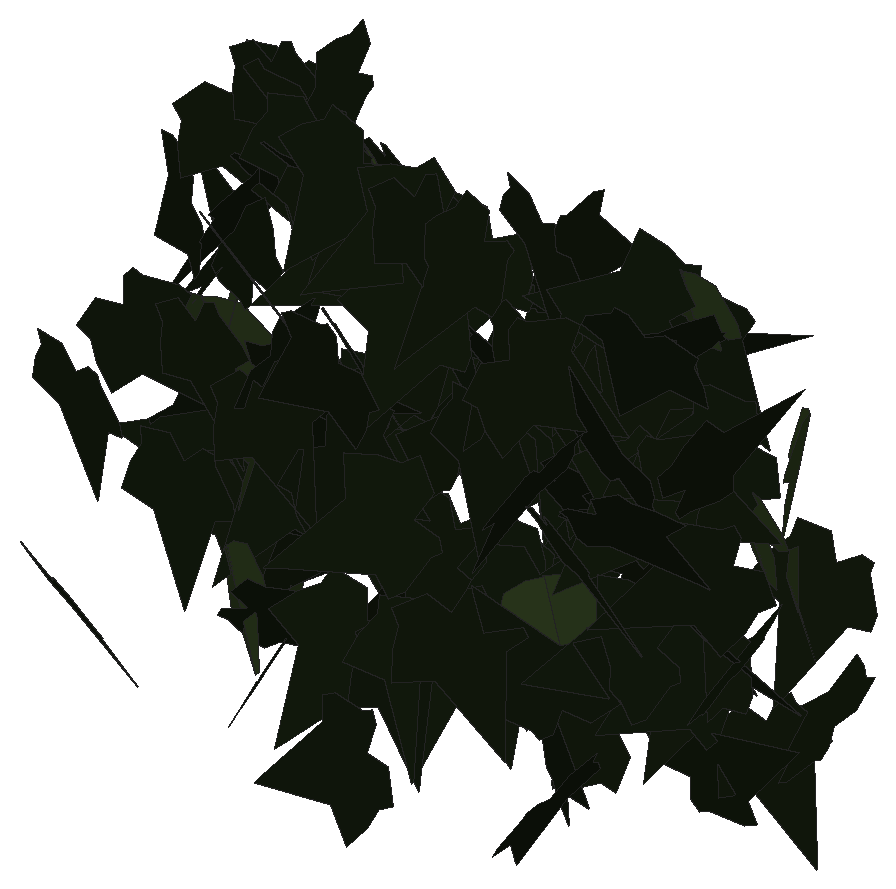
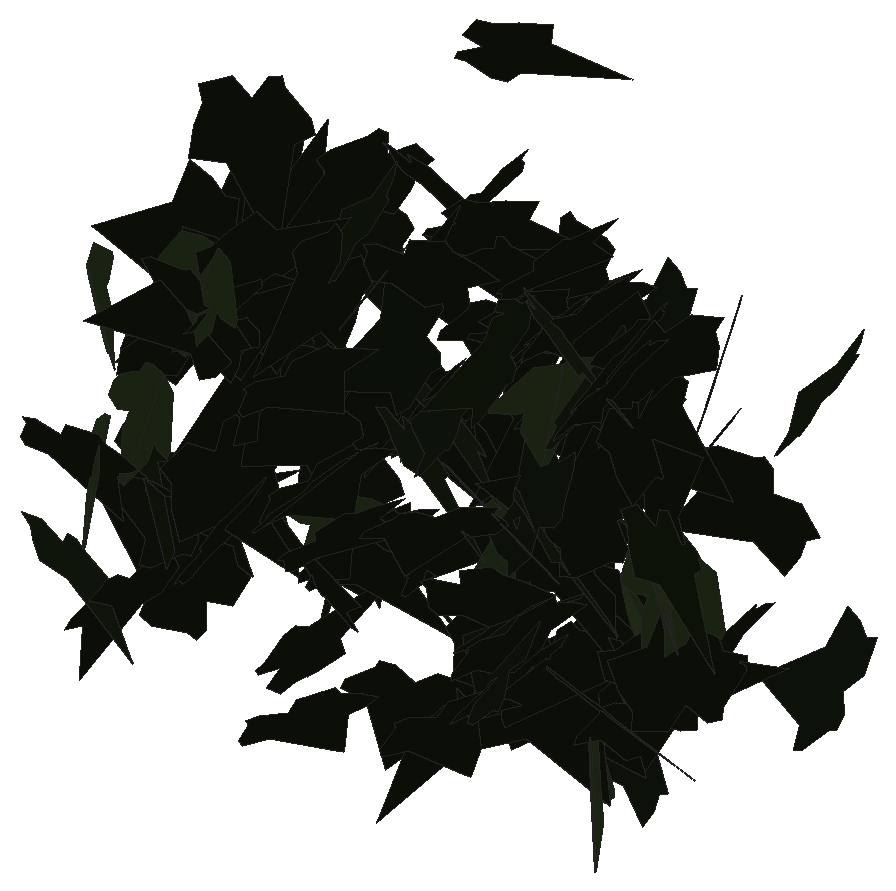
# SketchUp Ruby script. Lengths in inches.
U = 1.inch
M = Sketchup.active_model
def pt(a) = Geom::Point3d.new(a.map { |v| v * U })
def face(e, loops, mat)
  f = e.add_face(loops[0].map { |a| pt(a) })
  loops[1..].each { |l| e.add_face(l.map { |a| pt(a) }).erase! }
  f.material = f.back_material = mat if mat
  f
end
# faces: each face lists its corners as indices into pts; further lists are holes
def faces(e, pts, list, mat = nil) = list.each { |f| face(e, (f[0].is_a?(Array) ? f : [f]).map { |l| l.map { |i| pts[i] } }, mat) }
# xy, xz, yz: faces in a plane at the given z, y or x. An outline is a flat list of corners, or four numbers for a rectangle; further outlines are holes
def ring(l) = l.size == 4 ? [[l[0], l[1]], [l[2], l[1]], [l[2], l[3]], [l[0], l[3]]] : l.each_slice(2).to_a
def flat(e, list, mat, &to3) = list.each { |f| face(e, (f[0].is_a?(Array) ? f : [f]).map { |l| ring(l).map { |u, v| to3.(u, v) } }, mat) }
def xy(e, z, list, mat = nil) = flat(e, list, mat) { |x, y| [x, y, z] }
def xz(e, y, list, mat = nil) = flat(e, list, mat) { |x, z| [x, y, z] }
def yz(e, x, list, mat = nil) = flat(e, list, mat) { |y, z| [x, y, z] }
def lines(e, pts, list) = list.each { |a, b| e.add_line(pt(pts[a]), pt(pts[b])) }
# prism: a flat outline (further loops are holes) pulled along v
def prism(e, loops, v, mat = nil)
  f = face(e, loops, mat); d = Geom::Vector3d.new(v.map { |x| x * U })
  f.pushpull(f.normal.samedirection?(d) ? d.length : -d.length)
end
def box(e, o, s, mat = nil) = prism(e, [[o, [o[0] + s[0], o[1], o[2]], [o[0] + s[0], o[1] + s[1], o[2]], [o[0], o[1] + s[1], o[2]]]], [0, 0, s[2]], mat)
def at(x, y, z, deg = 0) = Geom::Transformation.translation(pt([x, y, z])) * Geom::Transformation.rotation(ORIGIN, Z_AXIS, deg.degrees)
def axes(o, x, y, z) = Geom::Transformation.new([*x, 0, *y, 0, *z, 0, *pt(o).to_a, 1])
def part(name) = M.definitions.add(name)
# library, detail: a bought-in or finely detailed component or shape, given as its bounding box
def library(name, o, s) = part(name).tap { |d| box(d.entities, o, s) }
def detail(e, o, s) = box(e.add_group.entities, o, s)
def put(e, d, t, mat = nil) = e.add_instance(d, t).tap { |i| i.material = mat if mat }
def group(e, t, mat = nil) = e.add_group.tap { |g| g.transformation = t; g.material = mat if mat }.entities
root = M.entities
M.materials.add("efeu1").color = [18, 25, 13]
M.materials.add("efeu2").color = [43, 57, 29]
c1 = part("ivyleaf_9")
p = [[1.54,2.16,1.25],[1.36,2.04,1.19],[-0.21,0.99,0.68],[-0.71,1.11,0.82],[-0.85,0.86,0.67],[-0.8,0.17,0.21],
  [-0.9,-0.01,0.1],[-0.67,-0.16,-0.02],[-0.08,-0.08,-0.05],[-0.03,-0.6,-0.4],[0.65,-0.88,-0.66],[0.83,-0.6,-0.49],
  [1.29,-0.42,-0.43],[1.8125,-0.07,-0.26],[1.21,0.44,0.15]]
faces(c1.entities,p,[[0,1,2,3,4,5,6,7,8,9,10,11,12,13,14]],"efeu1")
c2 = part("ivyleaf_10")
p = [[0,0.5,-0.03],[-0.0625,2.02,-0.43],[-0.19,2.01,-0.46],[-0.54,1.05,-0.29],[-0.52,0.625,-0.18],[-0.83,0.76,-0.28],
  [-1.16,0.64,-0.33],[-1.15,0.33,-0.24],[-0.77,-0.39,0.02],[-0.3,-0.51,0.16],[0.04,-0.48,0.23],[-0.02,2.01,-0.4375],
  [-0.06,2.01,-0.43],[0.04,-0.49,0.23],[0.67,-0.49,0.14],[1.38,0.36,-0.2],[1.375,0.51,-0.24],[0.81,0.65,-0.19],
  [0.62,0.59,-0.15],[0.6,1.09,-0.28],[0.5,1.23,-0.31]]
faces(c2.entities,p,[[0,1,2,3,4,5,6,7,8,9,10],[11,12,0,13,14,15,16,17,18,19,20]],"efeu2")
put(root,c1,axes([51.35,215.87,253.11],[-0.41145,-0.092,0.26878],[-0.24884,-0.11152,-0.4191],[0.13706,-0.47864,0.04598]))
put(root,c1,axes([50.625,216.07,250.18],[0.07533,-0.3424,-0.35649],[0.1349,-0.33267,0.34804],[-0.47553,-0.14862,0.04227]))
put(root,c1,axes([45.79,217.7,251.95],[0.13272,-0.43587,0.20593],[0.08102,-0.19038,-0.45518],[0.47521,0.15419,0.0201]))
put(root,c1,axes([49.52,218.01,250.15],[-0.21924,-0.16792,-0.41682],[0.41987,0.08873,-0.25659],[0.16014,-0.46252,0.10211]))
put(root,c1,axes([51.6,217.75,249.28],[-0.128,0.47895,-0.06501],[0.01692,-0.06277,-0.49576],[-0.48304,-0.12911,-0.00014]))
put(root,c1,axes([50.28,217.91,250.75],[-0.1909,-0.23992,-0.39497],[0.27126,0.28779,-0.30592],[0.37413,-0.33108,0.02028]))
put(root,c1,axes([49.88,218.1,250.37],[-0.23688,-0.42136,-0.12785],[0.05294,0.11687,-0.48326],[0.43713,-0.24248,-0.01075]))
put(root,c1,axes([45.15,218.2,249.2],[0.28896,-0.315,0.25938],[0.20109,-0.16663,-0.42638],[0.35506,0.35072,0.03039]))
put(root,c1,axes([52.08,217.96,252.49],[0.46557,0.173,0.05758],[0.05322,0.02208,-0.49667],[-0.17439,0.4686,0.00214]))
put(root,c1,axes([48.71,218.47,249.89],[-0.38739,-0.31374,0.03864],[-0.02856,-0.02612,-0.4985],[0.31482,-0.38844,0.00232]))
put(root,c1,axes([51.29,218.27,250],[0.18488,0.0292,0.46364],[-0.45548,0.10956,0.17473],[-0.09139,-0.48697,0.06711]))
put(root,c1,axes([51.23,218.27,251.86],[0.39203,-0.29563,0.09439],[0.07771,-0.05372,-0.49099],[0.30045,0.39964,0.00382]))
put(root,c1,axes([48.59,218.2,252.85],[0.05868,0.09487,-0.4874],[-0.44445,-0.20881,-0.09416],[-0.22141,0.4443,0.05983]))
put(root,c1,axes([50.98,218.34,252.39],[-0.21451,0.39853,-0.21251],[0.07623,-0.19994,-0.4519],[-0.44517,-0.22627,0.02502]))
put(root,c1,axes([47.49,218.48,252.02],[-0.16949,-0.19347,-0.42877],[0.37457,0.22018,-0.24742],[0.28455,-0.40508,0.0703]))
put(root,c1,axes([51.81,219.0625,250.46],[-0.22661,-0.18803,0.40409],[-0.27736,-0.29536,-0.29298],[0.34888,-0.35694,0.02956]))
put(root,c1,axes([50.51,218.57,253.37],[0.146,-0.16701,-0.4481],[-0.04575,0.46149,-0.18691],[0.47602,0.09558,0.11948]))
put(root,c2,axes([46.71,219.04,249.54],[-0.32298,0.21802,-0.31328],[0.18804,-0.26624,-0.37915],[-0.33214,-0.36274,0.08999]))
put(root,c1,axes([48.16,218.65,251.5625],[0.08632,-0.15034,-0.46899],[-0.10738,0.45893,-0.16688],[0.48064,0.12953,0.04694]))
put(root,c1,axes([46.6,219.12,252.95],[0.30263,-0.30306,0.25802],[0.1881,-0.17676,-0.42823],[0.35076,0.35625,0.00702]))
put(root,c1,axes([47.13,218.76,249.375],[0.4439,0.08899,0.2122],[0.20749,0.04454,-0.45273],[-0.09948,0.49,0.00262]))
put(root,c1,axes([48.92,219.21,253.2],[-0.43249,-0.23725,-0.08163],[0.08064,0.0226,-0.49294],[0.23758,-0.43955,0.01871]))
put(root,c1,axes([51.34,219.11,252.21],[0.35604,-0.27321,0.22044],[-0.14764,0.16832,0.44707],[-0.31849,-0.38344,0.03918]))
put(root,c1,axes([50.75,218.8,249.26],[0.2778,-0.09382,-0.405],[-0.37079,0.16435,-0.29241],[0.188,0.4628,0.02174]))
put(root,c1,axes([52.45,219.43,251.4],[-0.06396,-0.07802,-0.48972],[-0.07238,-0.48702,0.08704],[-0.49058,0.08203,0.051]))
put(root,c1,axes([46.04,219.26,251.9],[0.21344,-0.45099,-0.03238],[-0.01382,0.02928,-0.49895],[0.45194,0.21389,0.00003]))
put(root,c1,axes([49.46,219.34,253.96],[-0.48359,-0.02923,-0.12363],[0.12572,-0.04015,-0.48227],[0.01827,-0.49753,0.04618]))
put(root,c1,axes([47.34,218.8125,252.22],[-0.01408,0.00747,-0.49975],[-0.27521,0.41721,0.01399],[0.41721,0.27546,-0.00764]))
put(root,c1,axes([51.68,219.12,253.79],[0.25871,0.20392,-0.37615],[-0.32707,-0.18914,-0.32749],[-0.27585,0.4155,0.03552]))
put(root,c1,axes([45.18,219.25,251.8],[0.00751,-0.108,-0.48814],[0.38155,0.3167,-0.0642],[0.32305,-0.37153,0.08717]))
put(root,c1,axes([45.62,219.57,250.07],[0.04433,-0.49397,0.06346],[-0.00286,-0.06396,-0.49588],[0.49802,0.0436,-0.0085]))
put(root,c1,axes([45.56,219.73,252.9],[-0.01251,-0.15168,0.47627],[-0.00523,-0.47636,-0.15185],[0.49982,-0.00879,0.01033]))
put(root,c1,axes([48.63,219.68,253.78],[-0.40534,-0.18395,0.22773],[-0.1835,-0.1434,-0.44245],[0.22809,-0.44227,0.04874]))
put(root,c1,axes([51.41,219.69,251.8125],[-0.3705,-0.30381,0.14293],[-0.10362,-0.099,-0.47902],[0.31936,-0.38458,0.0104]))
put(root,c1,axes([48.56,219.49,254.05],[0.16653,-0.45456,-0.12507],[-0.03282,0.12115,-0.48399],[0.47031,0.16941,0.01051]))
put(root,c1,axes([46.94,219.1,248.4],[-0.22982,0.34518,-0.27935],[-0.17475,0.21886,0.4142],[0.40822,0.28802,0.02004]))
put(root,c2,axes([47.75,219.375,250.62],[-0.33331,-0.10516,-0.35756],[0.33882,0.11432,-0.34947],[0.15525,-0.47526,-0.00494]))
put(root,c1,axes([46.91,219.7,250.47],[-0.48914,-0.05223,-0.08951],[0.08888,0.01062,-0.49192],[0.05329,-0.49715,-0.00111]))
put(root,c1,axes([48.25,219.63,249.53],[-0.12198,0.35546,-0.3298],[0.11397,-0.30953,-0.37577],[-0.47131,-0.16685,-0.00551]))
put(root,c1,axes([48.67,219.91,250.25],[-0.10298,-0.45661,0.17579],[-0.03356,-0.17263,-0.46805],[0.48813,-0.1082,0.00491]))
put(root,c1,axes([49.11,219.93,251.53],[0.04766,-0.46724,0.17151],[0.00392,-0.17194,-0.46949],[0.49771,0.0461,-0.01273]))
put(root,c1,axes([47.4375,220.01,253.85],[-0.20116,-0.39386,0.23326],[-0.04898,-0.23481,-0.43871],[0.45512,-0.19935,0.05588]))
put(root,c1,axes([49.13,219.43,251.54],[-0.23701,0.36643,0.24404],[-0.17224,0.17789,-0.43438],[-0.40517,-0.28997,0.0419]))
put(root,c1,axes([51.65,220.05,249.71],[-0.25432,-0.26486,0.33936],[-0.13242,-0.32692,-0.35439],[0.40962,-0.27014,0.09614]))
put(root,c2,axes([50.05,219.65,250.08],[0.41617,0.23492,0.14703],[0.10438,0.11288,-0.47578],[-0.25673,0.4267,0.04491]))
put(root,c2,axes([46.31,219.93,250.61],[0.24468,-0.38467,0.20532],[0.11109,-0.17268,-0.4559],[0.42165,0.26872,0.00097]))
put(root,c1,axes([48.73,219.51,249.07],[-0.2026,0.31297,0.33317],[-0.21295,0.25785,-0.37171],[-0.40448,-0.29251,0.02881]))
put(root,c1,axes([52.01,219.41,252.18],[0.1162,0.0072,0.48626],[0.32444,0.37128,-0.08302],[-0.36227,0.33481,0.08161]))
put(root,c1,axes([49.68,219.97,250.0625],[-0.10268,-0.48582,-0.05862],[0.00488,0.05888,-0.4965],[0.48932,-0.10253,-0.00735]))
put(root,c1,axes([47.82,220.0625,253.04],[-0.43186,-0.0976,0.23231],[-0.19799,-0.15371,-0.43264],[0.15587,-0.46567,0.09411]))
put(root,c1,axes([47.86,219.92,253.2],[-0.14804,-0.43173,-0.20419],[0.07395,0.19048,-0.45634],[0.47182,-0.16532,0.00746]))
put(root,c1,axes([51.34,219.59,251.93],[0.10364,-0.07318,-0.48364],[0.1333,0.47989,-0.04405],[0.47063,-0.1198,0.11898]))
put(root,c1,axes([51.7,219.87,248.67],[0.02901,-0.03657,0.49782],[0.44078,-0.23214,-0.04274],[0.23425,0.44133,0.01877]))
put(root,c1,axes([47.22,219.82,250.99],[-0.08668,0.43153,-0.23722],[0.0497,-0.23197,-0.44014],[-0.48992,-0.09988,-0.00268]))
put(root,c1,axes([49.57,220.17,250.1],[-0.15482,-0.46758,0.08603],[-0.02918,-0.08096,-0.49254],[0.47453,-0.15753,-0.00222]))
put(root,c1,axes([49.55,219.96,252.83],[0.23815,-0.43423,-0.06876],[-0.02479,0.06481,-0.49516],[0.43894,0.23926,0.00934]))
put(root,c1,axes([49.66,220.08,249.9],[-0.47687,-0.14973,0.01325],[-0.0123,-0.00508,-0.49982],[0.14981,-0.47703,0.00116]))
put(root,c1,axes([46.67,219.82,251.28],[0.28434,-0.09284,0.40066],[0.39574,-0.07086,-0.29727],[0.11197,0.48617,0.03319]))
put(root,c1,axes([48.96,220.1,253.48],[-0.42133,-0.2545,-0.08778],[0.06661,0.0594,-0.49197],[0.26084,-0.42626,-0.01615]))
put(root,c1,axes([48.99,219.87,252.48],[0.45557,-0.17222,0.11312],[0.10166,-0.05088,-0.4869],[0.17922,0.46664,-0.01134]))
put(root,c1,axes([50.72,219.625,251.36],[0.42662,0.19616,0.17181],[0.14045,0.10472,-0.4683],[-0.21971,0.44783,0.03425]))
put(root,c1,axes([47.51,219.97,251.125],[-0.42116,0.26543,-0.04662],[0.03965,-0.02452,-0.49782],[-0.26656,-0.42302,-0.0004]))
put(root,c1,axes([50.08,219.85,251.3125],[0.47623,-0.04409,0.14582],[0.14478,-0.01783,-0.47825],[0.04737,0.49773,-0.00421]))
put(root,c1,axes([50.35,220.25,248.56],[-0.08063,-0.47757,-0.1242],[0.01738,-0.12852,0.48289],[-0.49315,0.07355,0.03732]))
put(root,c1,axes([51.65,220.21,249.9],[-0.44803,-0.17396,-0.13786],[0.14922,-0.00618,-0.47717],[0.16431,-0.46872,0.05745]))
put(root,c1,axes([52.22,219.73,249.97],[-0.04694,0.42165,0.26459],[-0.0782,0.25622,-0.42218],[-0.49161,-0.08102,0.0419]))
put(root,c1,axes([46.95,219.97,253.59],[0.3,-0.29696,-0.26798],[-0.04319,0.30897,-0.39073],[0.39766,0.25759,0.15973]))
put(root,c1,axes([49.36,220.43,253.66],[0.10811,-0.3971,0.28394],[0.09334,-0.26864,-0.41124],[0.47917,0.14193,0.01605]))
put(root,c1,axes([45.92,220.3125,249.67],[-0.12497,-0.47035,-0.11469],[0.03933,0.1082,-0.48657],[0.48253,-0.13063,0.00996]))
put(root,c1,axes([46.625,220.375,253.79],[-0.06753,-0.49509,-0.01816],[0.00248,0.01799,-0.49967],[0.49541,-0.06757,0.00003]))
put(root,c1,axes([47.03,220.28,249.73],[-0.00464,0.2605,-0.42675],[-0.09405,-0.41961,-0.25512],[-0.49105,0.07791,0.05289]))
put(root,c1,axes([45.89,220.34,249.9],[-0.18319,-0.02676,0.46446],[-0.46203,-0.04805,-0.185],[0.05454,-0.49697,-0.00713]))
put(root,c1,axes([45.92,220.37,252.95],[-0.24508,0.22557,-0.3729],[0.14309,-0.36245,-0.31329],[-0.41166,-0.26028,0.1131]))
put(root,c1,axes([51.48,220.3,249.87],[0.26014,-0.25828,0.34003],[0.29557,-0.17843,-0.36166],[0.30816,0.38917,0.05985]))
put(root,c1,axes([47.07,220.45,251.37],[0.39554,-0.17046,-0.25396],[0.24213,-0.07916,0.43024],[-0.18688,-0.46333,0.01993]))
put(root,c1,axes([47.3,220.38,250.17],[-0.02465,-0.49127,-0.08971],[0.11688,0.08165,-0.47924],[0.48552,-0.0446,0.11081]))
put(root,c1,axes([50.59,220.34,252.68],[-0.34152,-0.27178,-0.24392],[0.19435,0.14748,-0.43644],[0.30918,-0.39292,0.0049]))
put(root,c1,axes([46.23,220.05,253.42],[0.49201,0.01754,0.08727],[0.08726,0.00171,-0.49232],[-0.01757,0.49969,-0.00138]))
put(root,c1,axes([51.66,220.66,251.95],[-0.00171,-0.29976,-0.40018],[-0.00672,-0.40013,0.29975],[-0.49995,0.0064,-0.00266]))
put(root,c1,axes([47.99,220.52,252.27],[0.24136,-0.40084,0.17628],[0.09537,-0.14834,-0.46787],[0.42738,0.25947,0.00485]))
put(root,c1,axes([47.18,220.32,249.61],[0.01206,0.3798,-0.32497],[-0.2059,-0.29243,-0.34942],[-0.45548,0.14225,0.14935]))
put(root,c1,axes([45.66,220.29,253.84],[0.00781,-0.35252,-0.3545],[-0.02096,0.354,-0.35249],[0.4995,0.02037,-0.00925]))
put(root,c1,axes([45.23,220.49,250.08],[0.29855,0.26542,0.3007],[-0.23116,-0.19248,0.3994],[0.32777,-0.3775,0.00778]))
put(root,c1,axes([45.93,220.22,252.06],[0.03831,-0.03969,0.49695],[-0.28634,0.40625,0.05452],[-0.40809,-0.28877,0.0084]))
put(root,c1,axes([51,220.48,250.72],[-0.09905,0.34496,-0.34813],[0.01331,-0.35314,-0.35371],[-0.48991,-0.07934,0.06078]))
put(root,c1,axes([50.66,220.68,252.99],[-0.18742,-0.01493,0.4633],[-0.39767,-0.2516,-0.16898],[0.23818,-0.43183,0.08243]))
put(root,c1,axes([48.59,220.47,249.03],[-0.22318,-0.30624,-0.32621],[0.21709,0.24464,-0.37819],[0.39124,-0.31044,0.02376]))
put(root,c1,axes([48.79,220.32,251.66],[-0.34692,0.34916,0.08792],[-0.06917,0.05518,-0.49211],[-0.35336,-0.35361,0.01002]))
put(root,c2,axes([45.37,220.37,251.3125],[-0.48915,0.01802,-0.10203],[0.10206,-0.0009,-0.48947],[-0.01782,-0.49967,-0.00279]))
put(root,c1,axes([46.25,220.64,253.2],[0.22496,-0.41052,0.17568],[0.10725,-0.14128,-0.46748],[0.43346,0.24801,0.0245]))
put(root,c1,axes([47.73,220.66,251.56],[-0.47411,0.03337,-0.15526],[0.14787,-0.08549,-0.46992],[-0.05791,-0.49151,0.0712]))
put(root,c1,axes([50.83,220.9,249.95],[-0.11628,-0.32121,0.36511],[-0.06164,-0.36264,-0.33867],[0.48237,-0.12377,0.04474]))
put(root,c1,axes([52.05,220.56,249],[0.09831,-0.43292,-0.23003],[-0.05619,0.22312,-0.44392],[0.48701,0.11313,-0.00479]))
put(root,c2,axes([52.33,220.7,252.25],[0.27415,-0.40063,0.11973],[0.09638,-0.07877,-0.48426],[0.40688,0.2886,0.03403]))
put(root,c1,axes([50.54,220.77,252.6],[-0.12219,-0.47329,-0.10521],[0.03893,0.09857,-0.48864],[0.48327,-0.12761,0.01277]))
put(root,c1,axes([47.14,220.73,249.78],[0.11656,-0.46481,-0.14271],[0.00359,0.14757,-0.47771],[0.48621,0.11034,0.03774]))
put(root,c2,axes([46.69,220.625,253.14],[0.17161,0.46767,0.04282],[0.00256,0.04466,-0.498],[-0.46962,0.17114,0.01293]))
put(root,c2,axes([46.28,220.57,249.01],[0.1903,-0.3772,-0.26741],[-0.07825,0.25873,-0.42064],[0.4557,0.20195,0.03944]))
put(root,c1,axes([49.88,220.49,249.88],[-0.06177,0.21607,0.44665],[-0.2911,0.34872,-0.20894],[-0.4018,-0.28585,0.08271]))
put(root,c2,axes([45.3,220.89,251.67],[0.32113,-0.37209,0.09179],[0.05743,-0.07168,-0.49149],[0.37891,0.32621,-0.0033]))
put(root,c1,axes([45.68,220.875,253.93],[0.19078,-0.45729,-0.06702],[-0.02822,0.06084,-0.49548],[0.46131,0.19284,-0.0026]))
put(root,c1,axes([47.87,220.6875,249],[0.12655,-0.34166,-0.34243],[-0.03611,0.34629,-0.35886],[0.48237,0.11556,0.06298]))
put(root,c2,axes([51.64,220.73,251.28],[-0.44327,0.22525,-0.05269],[0.04945,-0.01898,-0.49719],[-0.22598,-0.44598,-0.00545]))
put(root,c1,axes([46.31,220.86,249.97],[-0.43997,0.19684,0.13296],[-0.15432,-0.02408,-0.47498],[-0.18059,-0.45899,0.08195]))
put(root,c1,axes([47.9375,220.96,251.3125],[-0.09267,-0.44711,-0.20372],[0.16493,0.16698,-0.44149],[0.46283,-0.14902,0.11653]))
put(root,c1,axes([47.125,220.875,253.38],[0.38982,-0.31033,0.04169],[0.03791,-0.01931,-0.49819],[0.31081,0.39157,0.00848]))
put(root,c1,axes([47.46,221.09,250.79],[-0.43533,-0.24547,0.01522],[-0.0115,-0.01058,-0.49976],[0.24567,-0.43547,0.00357]))
put(root,c1,axes([52.73,220.69,249.21],[-0.2441,0.40204,0.16966],[-0.15669,0.10068,-0.46402],[-0.40727,-0.2797,0.07684]))
put(root,c1,axes([52.4375,221.07,250.69],[-0.43353,-0.19302,-0.15747],[0.15582,0.03648,-0.4737],[0.19436,-0.4598,0.02852]))
put(root,c1,axes([49.31,221.17,251.35],[-0.15304,-0.47269,0.05605],[-0.02342,-0.05133,-0.49681],[0.47543,-0.15468,-0.00643]))
put(root,c1,axes([45.34,220.77,251.99],[-0.27197,0.41953,-0.00486],[0.00233,-0.00428,-0.49998],[-0.41956,-0.27198,0.00037]))
put(root,c1,axes([49.54,221.18,248.7],[-0.25255,-0.4307,0.02679],[0.02878,-0.04779,-0.49688],[0.43057,-0.24943,0.04893]))
put(root,c1,axes([46.91,221.13,250.1],[0.20482,-0.33589,0.30859],[0.15195,-0.26871,-0.39333],[0.43007,0.2549,-0.008]))
put(root,c2,axes([52.3,220.7,250.53],[-0.30049,0.3342,0.21913],[-0.16404,0.14685,-0.44891],[-0.36441,-0.34168,0.02139]))
put(root,c1,axes([49.5,220.53,253.375],[0.01066,0.06385,-0.49579],[-0.27157,0.41708,0.04788],[0.41969,0.26826,0.04357]))
put(root,c1,axes([45.67,221.16,253.68],[0.05229,-0.49458,0.0515],[0.00267,-0.0515,-0.49733],[0.49725,0.05229,-0.00275]))
put(root,c1,axes([49.34,221.25,251.25],[-0.0716,-0.47249,0.14704],[0.04876,-0.15459,-0.473],[0.49244,-0.05339,0.06821]))
put(root,c1,axes([46.54,221.04,254.07],[-0.45785,0.16191,-0.11899],[0.09885,-0.07628,-0.48416],[-0.17493,-0.46687,0.03784]))
put(root,c1,axes([49.48,221.31,252.51],[-0.21956,-0.44442,0.06548],[-0.01824,-0.06401,-0.49555],[0.44885,-0.21999,0.0119]))
put(root,c1,axes([50.66,220.7,252.59],[0.3287,0.06031,0.37191],[0.31375,0.22946,-0.3145],[-0.20861,0.44013,0.113]))
put(root,c1,axes([46.8,221.27,250.58],[-0.08932,-0.49191,0.00649],[-0.0007,-0.00647,-0.49996],[0.49196,-0.08932,0.00047]))
put(root,c1,axes([47.65,221.27,249.34],[-0.2042,-0.45465,-0.03989],[0.02152,0.03407,-0.49837],[0.45589,-0.20525,0.00565]))
put(root,c1,axes([50.72,221.09,252.76],[-0.05259,-0.16818,-0.46792],[0.42792,0.22432,-0.12872],[0.25322,-0.414,0.12034]))
put(root,c2,axes([50.74,221.03,253.16],[-0.47751,0.13692,-0.05691],[0.04182,-0.05973,-0.49465],[-0.14225,-0.47716,0.04559]))
put(root,c1,axes([48.98,221.44,250.9375],[-0.25768,-0.37265,0.2115],[-0.05208,-0.21773,-0.44708],[0.42531,-0.25244,0.0734]))
